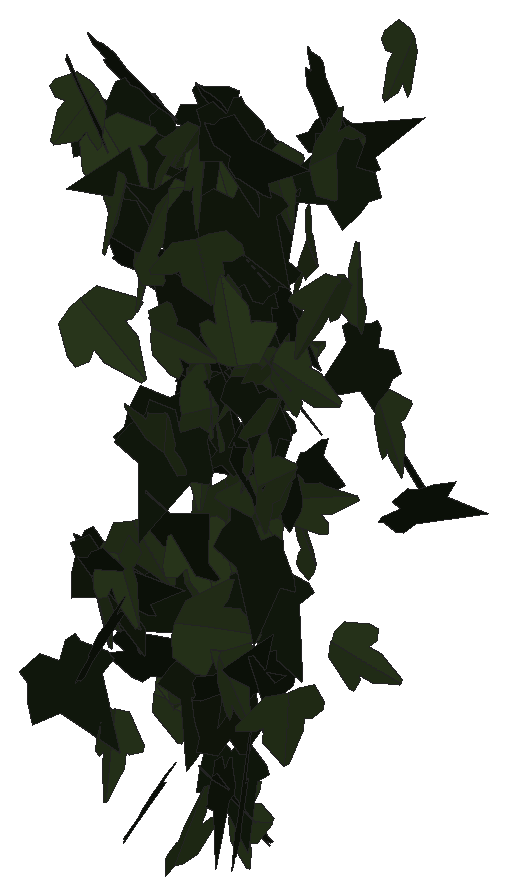
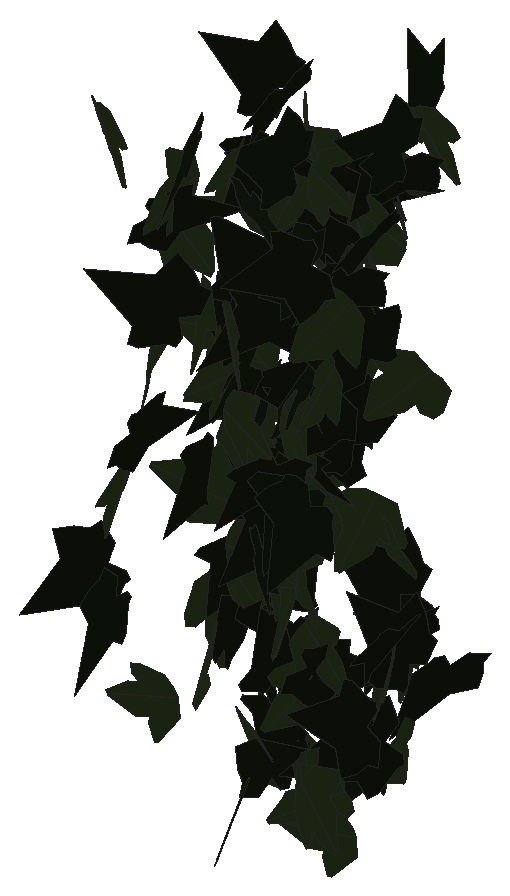
# SketchUp Ruby script. Lengths in inches.
U = 1.inch
M = Sketchup.active_model
def pt(a) = Geom::Point3d.new(a.map { |v| v * U })
def face(e, loops, mat)
  f = e.add_face(loops[0].map { |a| pt(a) })
  loops[1..].each { |l| e.add_face(l.map { |a| pt(a) }).erase! }
  f.material = f.back_material = mat if mat
  f
end
# faces: each face lists its corners as indices into pts; further lists are holes
def faces(e, pts, list, mat = nil) = list.each { |f| face(e, (f[0].is_a?(Array) ? f : [f]).map { |l| l.map { |i| pts[i] } }, mat) }
# xy, xz, yz: faces in a plane at the given z, y or x. An outline is a flat list of corners, or four numbers for a rectangle; further outlines are holes
def ring(l) = l.size == 4 ? [[l[0], l[1]], [l[2], l[1]], [l[2], l[3]], [l[0], l[3]]] : l.each_slice(2).to_a
def flat(e, list, mat, &to3) = list.each { |f| face(e, (f[0].is_a?(Array) ? f : [f]).map { |l| ring(l).map { |u, v| to3.(u, v) } }, mat) }
def xy(e, z, list, mat = nil) = flat(e, list, mat) { |x, y| [x, y, z] }
def xz(e, y, list, mat = nil) = flat(e, list, mat) { |x, z| [x, y, z] }
def yz(e, x, list, mat = nil) = flat(e, list, mat) { |y, z| [x, y, z] }
def lines(e, pts, list) = list.each { |a, b| e.add_line(pt(pts[a]), pt(pts[b])) }
# prism: a flat outline (further loops are holes) pulled along v
def prism(e, loops, v, mat = nil)
  f = face(e, loops, mat); d = Geom::Vector3d.new(v.map { |x| x * U })
  f.pushpull(f.normal.samedirection?(d) ? d.length : -d.length)
end
def box(e, o, s, mat = nil) = prism(e, [[o, [o[0] + s[0], o[1], o[2]], [o[0] + s[0], o[1] + s[1], o[2]], [o[0], o[1] + s[1], o[2]]]], [0, 0, s[2]], mat)
def at(x, y, z, deg = 0) = Geom::Transformation.translation(pt([x, y, z])) * Geom::Transformation.rotation(ORIGIN, Z_AXIS, deg.degrees)
def axes(o, x, y, z) = Geom::Transformation.new([*x, 0, *y, 0, *z, 0, *pt(o).to_a, 1])
def part(name) = M.definitions.add(name)
# library, detail: a bought-in or finely detailed component or shape, given as its bounding box
def library(name, o, s) = part(name).tap { |d| box(d.entities, o, s) }
def detail(e, o, s) = box(e.add_group.entities, o, s)
def put(e, d, t, mat = nil) = e.add_instance(d, t).tap { |i| i.material = mat if mat }
def group(e, t, mat = nil) = e.add_group.tap { |g| g.transformation = t; g.material = mat if mat }.entities
root = M.entities
M.materials.add("efeu1").color = [18, 25, 13]
M.materials.add("efeu2").color = [43, 57, 29]
c1 = part("ivyleaf_10")
p = [[0,0.5,-0.03],[-0.0625,2.02,-0.43],[-0.19,2.01,-0.46],[-0.54,1.05,-0.29],[-0.52,0.625,-0.18],[-0.83,0.76,-0.28],
  [-1.16,0.64,-0.33],[-1.15,0.33,-0.24],[-0.77,-0.39,0.02],[-0.3,-0.51,0.16],[0.04,-0.48,0.23],[-0.02,2.01,-0.4375],
  [-0.06,2.01,-0.43],[0.04,-0.49,0.23],[0.67,-0.49,0.14],[1.38,0.36,-0.2],[1.375,0.51,-0.24],[0.81,0.65,-0.19],
  [0.62,0.59,-0.15],[0.6,1.09,-0.28],[0.5,1.23,-0.31]]
faces(c1.entities,p,[[0,1,2,3,4,5,6,7,8,9,10],[11,12,0,13,14,15,16,17,18,19,20]],"efeu2")
c2 = part("ivyleaf_9")
p = [[1.54,2.16,1.25],[1.36,2.04,1.19],[-0.21,0.99,0.68],[-0.71,1.11,0.82],[-0.85,0.86,0.67],[-0.8,0.17,0.21],
  [-0.9,-0.01,0.1],[-0.67,-0.16,-0.02],[-0.08,-0.08,-0.05],[-0.03,-0.6,-0.4],[0.65,-0.88,-0.66],[0.83,-0.6,-0.49],
  [1.29,-0.42,-0.43],[1.8125,-0.07,-0.26],[1.21,0.44,0.15]]
faces(c2.entities,p,[[0,1,2,3,4,5,6,7,8,9,10,11,12,13,14]],"efeu1")
put(root,c1,axes([559.2,134.23,201.89],[-0.90264,0.06518,-0.56528],[0.56498,-0.02353,-0.90487],[-0.06774,-1.06478,-0.01461]))
put(root,c2,axes([559.28,132.69,203.625],[0.25324,-0.87405,-0.17808],[-0.05092,0.17065,-0.91],[0.89055,0.25831,-0.00139]))
put(root,c1,axes([559.92,129.47,205.62],[0.81318,-0.2449,-0.45148],[-0.43519,0.12051,-0.84921],[0.2728,0.92226,-0.00893]))
put(root,c1,axes([559.87,130.13,189.68],[-0.78884,0.53505,0.1537],[-0.14077,0.06618,-0.95288],[-0.5386,-0.80095,0.02394]))
put(root,c2,axes([559,133.31,188.48],[0.32829,0.13811,-0.87175],[0.77315,0.40363,0.35511],[0.42573,-0.83952,0.02732]))
put(root,c1,axes([559.79,134.66,186.5625],[0.19927,-0.95291,0.39518],[0.10577,-0.38149,-0.97323],[1.02616,0.22437,0.02358]))
put(root,c2,axes([559.45,131.17,190.35],[0.1662,-0.94323,-0.41182],[-0.03,0.41254,-0.95698],[1.02878,0.16441,0.03862]))
put(root,c1,axes([559.86,131.23,189.3],[-0.7234,0.72719,0.04566],[-0.03565,0.02894,-1.02572],[-0.72775,-0.72426,0.00487]))
put(root,c2,axes([559.16,131.2,189.6],[0.2261,-0.2889,0.97302],[0.73864,-0.6369,-0.36074],[0.69617,0.76958,0.06673]))
put(root,c2,axes([559.22,131.4375,205.74],[0.61256,-0.45712,0.56824],[0.47876,-0.30774,-0.76366],[0.55014,0.7768,0.03186]))
put(root,c1,axes([559.35,130.43,198.11],[0.66669,0.39586,0.80002],[0.67868,0.42377,-0.77526],[-0.57977,0.95128,0.01245]))
put(root,c1,axes([560.15,133.36,199.04],[0.00259,-0.38442,-0.8398],[0.05826,0.8382,-0.3835],[0.92176,-0.0519,0.0266]))
put(root,c2,axes([560.23,134.22,195.3],[0.23633,0.87871,0.40823],[0.12,0.39042,-0.90984],[-0.96145,0.26472,-0.01321]))
put(root,c2,axes([559.78,128.59,187.99],[0.19453,-0.72384,-0.70986],[-0.01042,0.72135,-0.7384],[1.01378,0.14631,0.12863]))
put(root,c2,axes([559.79,130.67,204.91],[-0.06111,-0.61134,-0.73367],[0.22775,0.70463,-0.60611],[0.92744,-0.21332,0.1005]))
put(root,c2,axes([560.03,136.72,195.01],[-0.45508,0.08926,-0.77845],[0.71985,-0.30794,-0.45613],[-0.30949,-0.8475,0.08375]))
put(root,c2,axes([559.95,132.875,202.16],[-0.12834,-0.59721,-0.69735],[0.17621,0.67502,-0.61051],[0.90106,-0.21707,0.02006]))
put(root,c2,axes([559.71,131.66,187.02],[0.87815,0.14103,0.51566],[0.51049,0.07319,-0.88937],[-0.15871,1.01572,-0.00751]))
put(root,c2,axes([560.57,134.16,195.72],[0.20857,0.8879,0.40846],[0.10461,0.39498,-0.91201],[-0.97173,0.2331,-0.01051]))
put(root,c1,axes([559.79,133.43,184.8125],[-0.11527,-0.08976,-0.936],[0.93267,-0.13076,-0.10232],[-0.1195,-0.93397,0.10429]))
put(root,c2,axes([559.99,134.55,203.21],[0.10734,0.13717,-0.89428],[0.57349,0.6862,0.17409],[0.69976,-0.58343,-0.0055]))
put(root,c1,axes([560.13,133.38,185.91],[0.32182,0.27061,0.85149],[0.60418,0.60083,-0.4193],[-0.65821,0.68382,0.03144]))
put(root,c2,axes([560.09,131.82,199.2],[1.04688,0.11403,-0.23279],[0.22833,0.05293,1.05272],[0.12273,-1.07114,0.02724]))
put(root,c1,axes([560.68,129.83,185.74],[-0.02447,0.87777,-0.46591],[0.0038,-0.46597,-0.87807],[-0.99375,-0.0234,0.00811]))
put(root,c2,axes([560.25,129.02,205.9],[0.1023,-0.36131,0.95831],[0.38488,-0.87892,-0.37247],[0.94909,0.39537,0.04775]))
put(root,c1,axes([560.34,129.97,204.33],[0.65033,0.43203,0.5737],[0.48608,0.30496,-0.78066],[-0.52868,0.81182,-0.01205]))
put(root,c2,axes([560.54,133.51,201.5625],[-0.03617,-0.70313,0.65646],[0.07205,-0.65706,-0.6998],[0.95924,0.02284,0.07732]))
put(root,c1,axes([560.74,132.86,193.93],[0.0051,0.27879,0.91595],[0.02905,0.9155,-0.27881],[-0.957,0.02927,-0.00358]))
put(root,c1,axes([560.97,133.25,186.375],[0.18392,-0.95221,-0.29135],[-0.00676,0.29508,-0.96866],[0.99577,0.17788,0.04724]))
put(root,c1,axes([561.67,132.28,189.85],[-0.57246,0.04027,0.78396],[-0.78311,-0.0966,-0.56687],[0.05445,-0.96591,0.08937]))
put(root,c2,axes([561.51,132.49,189.07],[-0.06593,-0.31972,-0.89004],[-0.17931,-0.8718,0.32644],[-0.92857,0.19104,0.00015]))
put(root,c1,axes([560.37,130.57,202.29],[0.45014,-0.25701,-1.03394],[1.01039,-0.25306,0.50279],[-0.33795,-1.09892,0.12603]))
put(root,c2,axes([561.71,130.83,203.53],[-0.15041,-0.38716,-0.88076],[-0.21227,-0.85613,0.41259],[-0.93839,0.25572,0.04784]))
put(root,c1,axes([561.87,135.34,198.12],[0.15713,-0.0854,-0.9413],[-0.77631,0.53265,-0.17791],[0.53914,0.79184,0.01816]))
put(root,c1,axes([561.21,129.3,203.2],[0.64112,-0.65683,0.09752],[0.06717,-0.07071,-0.91786],[0.66062,0.64463,-0.00131]))
put(root,c2,axes([561.54,136.19,185.37],[-0.02244,-0.66644,0.68137],[0.02031,0.68107,0.66681],[-0.95289,0.03021,-0.00183]))
put(root,c2,axes([561.47,127.8,189.27],[0.07768,0.5784,0.83399],[0.11517,0.826,-0.58359],[-1.00837,0.1389,-0.00241]))
put(root,c2,axes([560.97,134.77,196.61],[0.12626,-0.54117,-0.7389],[0.05334,0.74896,-0.53943],[0.91432,0.03104,0.1335]))
put(root,c1,axes([561.24,130.71,200.94],[0.67739,-0.66424,0.18482],[0.13311,-0.12824,-0.94872],[0.67651,0.69034,0.0016]))
put(root,c2,axes([560.8,129.56,190.5],[0.24109,-0.31901,0.88483],[0.83372,-0.35039,-0.35349],[0.43544,0.84751,0.18692]))
put(root,c1,axes([561.02,133.29,192.15],[0.43014,-0.26362,0.82798],[0.75085,-0.35223,-0.50222],[0.43735,0.86401,0.04788]))
put(root,c1,axes([561.0625,129.3,191.59],[0.66861,-0.0808,0.79441],[0.78141,-0.14706,-0.67263],[0.16436,1.02786,-0.03379]))
put(root,c1,axes([561.82,131.58,204.08],[0.12322,-0.74909,0.5757],[0.06238,-0.57286,-0.75874],[0.9427,0.13582,-0.02504]))
put(root,c1,axes([561.88,132.82,196.99],[0.22029,-0.89383,0.28163],[0.0629,-0.27456,-0.92056],[0.93503,0.22905,-0.00443]))
put(root,c1,axes([561.81,133.13,191.2],[-0.57688,0.82919,-0.27494],[0.1567,-0.22591,-1.01012],[-0.85941,-0.59778,0.00037]))
put(root,c1,axes([561.58,130,201.1875],[0.78369,-0.6692,-0.46399],[0.35058,-0.30397,1.03052],[-0.73499,-0.85852,-0.00319]))
put(root,c1,axes([561.93,129.44,192.61],[-0.84648,-0.36436,-0.32955],[0.30444,0.12624,-0.92156],[0.38559,-0.89955,0.00415]))
put(root,c1,axes([561.7,132.2,194.68],[0.9932,-0.30287,0.44265],[0.42911,-0.11015,-1.0382],[0.32177,1.08178,0.01822]))
put(root,c2,axes([561.2,131.78,197.6],[0.39598,0.27725,-1.01789],[0.83902,0.57633,0.48338],[0.63954,-0.92776,-0.00391]))
put(root,c2,axes([561.65,132.93,197.58],[0.30771,-0.69708,0.52633],[0.21737,-0.47936,-0.76196],[0.84598,0.37672,0.00434]))
put(root,c1,axes([562.28,132.7,192.68],[-0.18918,-0.92063,-0.22612],[0.06296,0.21787,-0.9397],[0.94589,-0.19863,0.01733]))
put(root,c2,axes([561.96,130.36,201.54],[-0.59813,-0.1485,0.98807],[0.99889,-0.06188,0.59539],[-0.02342,1.15335,0.15916]))
put(root,c2,axes([562.01,130.15,195.0625],[-0.18678,-0.10082,1.13534],[1.03454,0.46791,0.21175],[-0.47843,1.05116,0.01463]))
put(root,c2,axes([561.79,132.36,201.53],[0.78482,-0.52143,0.29815],[0.25546,-0.15422,-0.94217],[0.54362,0.82526,0.01231]))
put(root,c2,axes([562.96,132.04,195.27],[-0.94454,-0.17449,0.08848],[-0.0857,-0.02313,-0.96049],[0.17587,-0.94839,0.00715]))
put(root,c2,axes([562.78,128.35,184.41],[0.0198,0.67615,0.64512],[0.02342,0.64471,-0.67643],[-0.93425,0.03049,-0.00328]))
put(root,c1,axes([562.02,131.85,196.7],[0.56113,-0.29933,0.71909],[0.68285,-0.2373,-0.63163],[0.3747,0.88071,0.07421]))
put(root,c2,axes([562.92,130.77,198.84],[0.51915,-0.09717,0.82242],[-0.79268,0.22268,0.52669],[-0.23973,-0.94673,0.03947]))
put(root,c2,axes([562.25,132.625,193.75],[0.91775,0.25049,0.0307],[0.02828,0.01301,-0.95131],[-0.25077,0.91817,0.0051]))
put(root,c1,axes([562.79,135.75,189.46],[-0.56877,0.70129,0.19131],[0.10968,-0.15734,0.90284],[0.71859,0.57908,0.01362]))
put(root,c1,axes([562.53,131.09,187.65],[-0.60584,-0.36888,-0.63161],[0.54059,0.32663,-0.7093],[0.4927,-0.81196,0.00161]))
put(root,c1,axes([563.625,132.84,192.24],[0.13684,-0.05826,-1.04865],[-0.97675,0.38164,-0.14866],[0.38604,0.98628,-0.00442]))
put(root,c1,axes([562.88,130.38,196.39],[0.15767,-0.33656,-1.00353],[0.20777,1.0047,-0.30431],[1.03787,-0.15,0.21337]))
put(root,c1,axes([562.59,131.8,203.7],[0.77016,0.36223,0.37402],[0.3268,0.1836,-0.85073],[-0.40535,0.83626,0.02477]))
put(root,c1,axes([563.24,133.93,200.13],[0.45049,-0.58358,-0.58199],[-0.31149,0.4935,-0.73596],[0.76305,0.54599,0.04316]))
put(root,c2,axes([562.23,132.49,204.71],[0.61026,-0.48236,0.58631],[0.47915,-0.33882,-0.77747],[0.58893,0.77549,0.025]))
put(root,c2,axes([563.61,132.43,203.11],[-0.55205,0.73691,0.32359],[-0.20576,0.25013,-0.92065],[-0.77808,-0.58898,0.01387]))
put(root,c2,axes([563.31,129.32,196.16],[-0.93145,-0.41684,-0.35993],[0.32421,0.15662,-1.02042],[0.44519,-0.98621,-0.00992]))
put(root,c2,axes([562.99,131.9375,199.98],[0.09656,-0.20229,-1.02126],[-0.01071,1.0254,-0.20412],[1.04105,0.02931,0.09263]))
put(root,c2,axes([562.79,136.89,201.73],[0.1792,-0.12521,0.94889],[0.95077,0.13429,-0.16184],[-0.11005,0.95628,0.14697]))
put(root,c1,axes([563.24,128.69,196.09],[-0.9417,0.08484,0.47864],[0.45246,-0.22848,0.93069],[0.1777,1.03136,0.1668]))
put(root,c1,axes([563.42,129.45,182.9375],[0.16893,-1.03066,0.09364],[0.01928,0.09799,1.04384],[-1.03473,-0.16644,0.03473]))
put(root,c1,axes([563.17,130.46,204.52],[0.58984,-0.44215,0.64999],[0.53075,-0.37546,-0.73704],[0.57991,0.79337,0.01344]))
put(root,c1,axes([563.23,128.73,199.62],[-0.02242,-0.07069,0.94311],[0.93097,0.16452,0.03446],[-0.16659,0.92892,0.06566]))
put(root,c2,axes([563.95,130.11,188.52],[-0.77287,-0.4206,-0.38923],[0.35432,0.1629,-0.87958],[0.45041,-0.84988,0.02403]))
put(root,c1,axes([564.14,133.93,200.59],[0.32645,-0.72806,-0.74673],[-0.11478,0.75262,-0.78398],[1.03658,0.31263,0.14836]))
put(root,c2,axes([563.75,131.82,200.22],[-0.38077,-0.29723,0.91157],[0.87019,0.30469,0.46283],[-0.40257,0.93974,0.13826]))
put(root,c1,axes([564.11,132.125,190.88],[-0.11246,0.46146,0.98257],[0.15774,-0.9704,0.4738],[1.07402,0.19084,0.0333]))
put(root,c2,axes([564.05,134.44,205.72],[0.64521,-0.34861,-0.57771],[-0.50733,0.27636,-0.73337],[0.44486,0.82078,0.00155]))
put(root,c2,axes([563.85,130.86,205.81],[0.32457,-0.86849,-0.30593],[-0.12902,0.27829,-0.92689],[0.91172,0.34856,-0.02225]))
put(root,c2,axes([563.75,128.8,192.98],[-0.34253,-0.15034,1.01336],[0.71092,-0.80423,0.12099],[0.73763,0.7053,0.35397]))
put(root,c2,axes([564.26,137.77,192.58],[0.83946,-0.08773,-0.5078],[-0.50247,0.07603,-0.8438],[0.11435,0.97815,0.02004]))
put(root,c2,axes([563.96,132.23,197.61],[0.9208,-0.25463,-0.12738],[-0.1236,0.03093,-0.95535],[0.25649,0.92905,-0.00311]))
put(root,c1,axes([564.14,129.19,193.22],[0.69137,0.68912,0.2772],[0.19816,0.19386,-0.97616],[-0.71587,0.71921,-0.00249]))
put(root,c1,axes([564.58,128.7,202.85],[-0.67324,-0.77958,-0.18345],[0.11726,0.14112,-1.03004],[0.79224,-0.68337,-0.00343]))
put(root,c1,axes([564.6,132.12,197.21],[0.08691,-0.12552,1.04397],[-0.24489,1.01631,0.14259],[-1.02258,-0.25406,0.05458]))
put(root,c2,axes([564.23,130.59,185.76],[-0.46444,-0.29987,-0.73908],[0.69355,0.27053,-0.54559],[0.39389,-0.82991,0.0892]))
put(root,c2,axes([564.29,130.73,184.03],[0.92741,-0.50843,-0.01362],[0.01772,0.00399,1.05757],[-0.5083,-0.9275,0.01202]))
put(root,c2,axes([564.68,129.9375,186.92],[-0.35388,-0.51689,0.85583],[0.50189,0.69335,0.62628],[-0.86471,0.61396,0.01325]))
put(root,c1,axes([564.52,130.73,198.24],[-0.09729,-0.3833,-0.94649],[0.27671,0.90531,-0.39506],[0.98295,-0.29279,0.01753]))
put(root,c1,axes([564.58,132.13,203.91],[-0.26102,0.92977,0.09922],[-0.03228,0.09399,-0.9657],[-0.93449,-0.26294,0.00564]))
put(root,c1,axes([564.55,131.08,197.1],[0.1084,-0.56668,0.81481],[-0.04769,0.81573,0.57367],[-0.99135,-0.10121,0.06149]))
put(root,c1,axes([564.72,130.01,200.69],[-0.62211,0.76455,-0.06126],[0.03521,-0.05034,-0.98567],[-0.76619,-0.62309,0.00445]))
put(root,c2,axes([564.38,130.54,203.47],[-0.26522,-0.36564,-0.8787],[0.4813,0.73541,-0.45128],[0.82106,-0.5492,-0.01929]))
put(root,c2,axes([564.56,129.79,185.63],[-0.4408,0.00348,-0.78847],[0.77881,-0.13913,-0.43602],[-0.12312,-0.89255,0.06489]))
put(root,c1,axes([565.13,134.88,198.41],[-0.12916,0.63905,-0.68012],[-0.19937,0.65186,0.65036],[0.91171,0.23308,0.04587]))
put(root,c1,axes([565.05,133.65,203.63],[-0.02048,0.12056,1.09236],[-0.39396,1.01913,-0.11986],[-1.02595,-0.39375,0.02422]))
put(root,c2,axes([564.83,132,196.35],[-0.12561,-0.46272,0.84173],[-0.26412,-0.79953,-0.47894],[0.92351,-0.2916,-0.02249]))
put(root,c2,axes([565.23,134.67,203.05],[-0.00237,-0.43186,-0.83523],[-0.04523,-0.83421,0.43147],[-0.93919,0.04126,-0.01867]))
put(root,c2,axes([564.33,132.58,199.09],[0.29252,-0.18727,-0.87388],[0.89315,0.09395,0.27884],[0.03177,-0.91674,0.20709]))
put(root,c2,axes([564.75,131.06,191.11],[-0.19662,-0.63344,-0.76609],[0.2416,0.72707,-0.66318],[0.96425,-0.31134,0.00995]))
put(root,c2,axes([565.25,132.22,194.24],[-0.01387,0.03621,-0.93856],[-0.54176,0.76647,0.03757],[0.76726,0.54186,0.00957]))
put(root,c2,axes([564.86,130.6,195.12],[-0.21124,-0.0947,1.08472],[0.08486,-1.10301,-0.07977],[1.08553,0.06779,0.21731]))
put(root,c2,axes([565.14,135.8,196.71],[0.11585,-0.36386,-0.85317],[0.34075,-0.78298,0.38019],[-0.86266,-0.35814,0.0356]))
put(root,c1,axes([565.4,130.58,194.61],[-0.18044,-0.94428,0.55322],[-0.09345,-0.54535,-0.96132],[1.0904,-0.203,0.00916]))
put(root,c1,axes([565.3,129.07,189.52],[-0.34736,0.89838,0.34334],[-0.13731,0.31498,-0.9631],[-0.9519,-0.37326,0.01364]))
put(root,c2,axes([564.86,129.41,188.57],[0.66416,0.72675,0.15353],[-0.10817,-0.10913,0.9845],[0.73488,-0.67289,0.00616]))
put(root,c1,axes([564.74,130.33,184.05],[0.20835,-0.37853,-0.86078],[0.70833,-0.5167,0.39867],[-0.61847,-0.71929,0.16661]))
put(root,c2,axes([564.95,130.85,197.33],[0.17974,-0.9474,0.35065],[0.08857,-0.34001,-0.96405],[1.00632,0.19914,0.02222]))
put(root,c1,axes([565.61,129.02,199.98],[0.92208,0.17737,0.33075],[-0.32906,-0.03982,0.93874],[0.18048,-0.9788,0.02174]))
put(root,c1,axes([565.27,127.6,191.54],[0.1771,0.37383,1.08122],[0.08849,1.08635,-0.3901],[-1.1406,0.14232,0.13761]))
put(root,c1,axes([565.52,130.58,197.06],[0.31543,-0.95193,0.48554],[0.16085,-0.45819,-1.0028],[1.05643,0.35399,0.00771]))
put(root,c2,axes([565.47,131.28,187.96],[-0.03867,0.24922,1.07237],[-0.32431,-1.028,0.22721],[1.0521,-0.30772,0.10945]))
put(root,c2,axes([564.77,129.99,205.3],[0.31632,-0.17335,0.9208],[0.80073,-0.45466,-0.36067],[0.48656,0.86093,-0.00507]))
put(root,c1,axes([564.96,132.41,193.33],[-0.22616,-0.30676,0.88598],[0.79365,0.42261,0.34891],[-0.49919,0.81088,0.15333]))
put(root,c1,axes([565.15,134.55,187.78],[-0.26327,0.0019,-0.89513],[0.87833,-0.17937,-0.25871],[-0.17261,-0.91564,0.04882]))
put(root,c1,axes([565.77,135.49,194.96],[-0.25811,0.89152,0.14434],[-0.04751,0.1365,-0.92811],[-0.90188,-0.26234,0.00759]))
put(root,c1,axes([565.98,136.05,206.51],[0.77575,-0.56855,-0.25553],[-0.19824,0.16173,-0.96171],[0.59097,0.80058,0.01282]))
put(root,c1,axes([565.39,131.64,198.01],[-0.20709,-0.01153,-0.95363],[0.91253,-0.28603,-0.19471],[-0.27719,-0.933,0.07148]))
put(root,c2,axes([566.53,127.93,185.08],[0.06556,0.00613,1.16954],[-0.0641,1.16963,-0.00254],[-1.16779,-0.06386,0.0658]))
put(root,c1,axes([566.43,129.17,195.88],[0.25497,-0.30388,-1.02495],[0.00209,1.05383,-0.31193],[1.06904,0.07042,0.24507]))
put(root,c2,axes([566.27,135.69,192.12],[0.61504,0.50332,0.51748],[0.37758,0.35512,-0.79417],[-0.61526,0.72107,0.02992]))
put(root,c1,axes([566.75,129.88,188.6],[-0.46805,-0.97271,-0.03245],[0.03054,0.02131,-1.07931],[0.97277,-0.46869,0.01827]))
put(root,c1,axes([566.79,131.73,200.9],[-0.06203,-0.85719,0.53445],[0.00599,-0.53576,-0.8586],[1.01014,-0.04946,0.03791]))
put(root,c2,axes([566.34,129.18,193.87],[0.07389,-1.03369,0.34224],[0.04267,-0.34001,-1.03619],[1.08804,0.08354,0.01739]))
